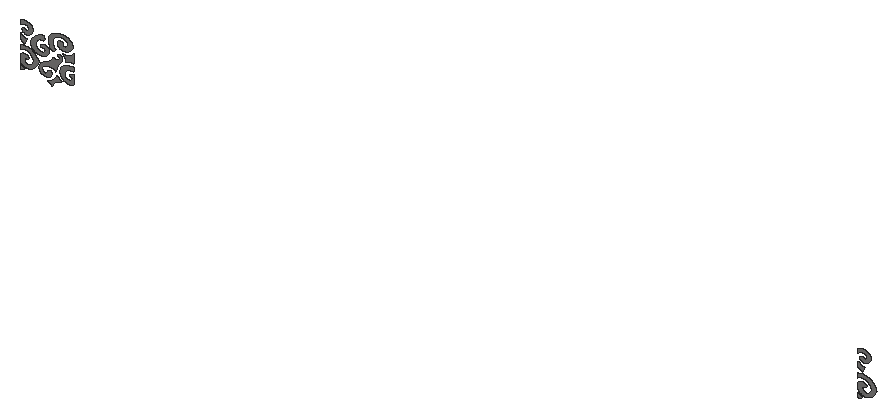
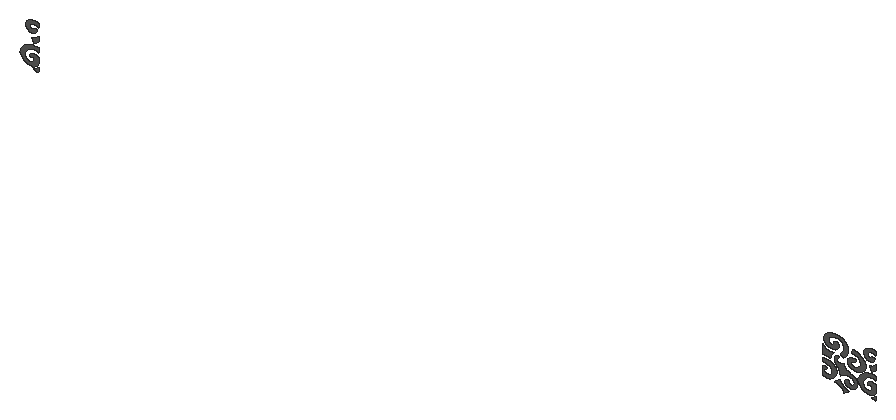
# SketchUp Ruby script. Lengths in inches.
U = 1.inch
M = Sketchup.active_model
def pt(a) = Geom::Point3d.new(a.map { |v| v * U })
def face(e, loops, mat)
  f = e.add_face(loops[0].map { |a| pt(a) })
  loops[1..].each { |l| e.add_face(l.map { |a| pt(a) }).erase! }
  f.material = f.back_material = mat if mat
  f
end
# faces: each face lists its corners as indices into pts; further lists are holes
def faces(e, pts, list, mat = nil) = list.each { |f| face(e, (f[0].is_a?(Array) ? f : [f]).map { |l| l.map { |i| pts[i] } }, mat) }
# xy, xz, yz: faces in a plane at the given z, y or x. An outline is a flat list of corners, or four numbers for a rectangle; further outlines are holes
def ring(l) = l.size == 4 ? [[l[0], l[1]], [l[2], l[1]], [l[2], l[3]], [l[0], l[3]]] : l.each_slice(2).to_a
def flat(e, list, mat, &to3) = list.each { |f| face(e, (f[0].is_a?(Array) ? f : [f]).map { |l| ring(l).map { |u, v| to3.(u, v) } }, mat) }
def xy(e, z, list, mat = nil) = flat(e, list, mat) { |x, y| [x, y, z] }
def xz(e, y, list, mat = nil) = flat(e, list, mat) { |x, z| [x, y, z] }
def yz(e, x, list, mat = nil) = flat(e, list, mat) { |y, z| [x, y, z] }
def lines(e, pts, list) = list.each { |a, b| e.add_line(pt(pts[a]), pt(pts[b])) }
# prism: a flat outline (further loops are holes) pulled along v
def prism(e, loops, v, mat = nil)
  f = face(e, loops, mat); d = Geom::Vector3d.new(v.map { |x| x * U })
  f.pushpull(f.normal.samedirection?(d) ? d.length : -d.length)
end
def box(e, o, s, mat = nil) = prism(e, [[o, [o[0] + s[0], o[1], o[2]], [o[0] + s[0], o[1] + s[1], o[2]], [o[0], o[1] + s[1], o[2]]]], [0, 0, s[2]], mat)
def at(x, y, z, deg = 0) = Geom::Transformation.translation(pt([x, y, z])) * Geom::Transformation.rotation(ORIGIN, Z_AXIS, deg.degrees)
def axes(o, x, y, z) = Geom::Transformation.new([*x, 0, *y, 0, *z, 0, *pt(o).to_a, 1])
def part(name) = M.definitions.add(name)
# library, detail: a bought-in or finely detailed component or shape, given as its bounding box
def library(name, o, s) = part(name).tap { |d| box(d.entities, o, s) }
def detail(e, o, s) = box(e.add_group.entities, o, s)
def put(e, d, t, mat = nil) = e.add_instance(d, t).tap { |i| i.material = mat if mat }
def group(e, t, mat = nil) = e.add_group.tap { |g| g.transformation = t; g.material = mat if mat }.entities
root = M.entities
M.materials.add("[0043_SaddleBrown]4").color = [124, 123, 122]
xz(root,589.17,[[416.17,173.83,415.69,174.24,415.1875,174.64,414.66,175.02,414.12,175.39,413.5625,175.74,412.98,176.08,412.39,176.4,411.78,176.71,411.15,177,410.51,177.27,409.85,177.53,409.1875,177.77,410.75,178.34,412.25,178.99,413.6875,179.72,415.05,180.52,416.32,181.39,417.51,182.32,418.6,183.31,419.6,184.35,420.48,185.44,421.26,186.58,421.93,187.75,422.47,188.95,423.02,188.49,423.58,188.03,424.74,187.15,425.33,186.72,425.93,186.29,426.54,185.87,427.16,185.46,427.79,185.06,428.43,184.66,429.07,184.27,429.73,183.89,428.07,183.57,426.46,183.14,424.92,182.59,423.45,181.94,422.09,181.19,420.83,180.35,419.7,179.42,418.69,178.41,417.83,177.34,417.12,176.21,416.56,175.04],[367.98,179.89,367.98,185.26,368.39,184.92,368.83,184.6,369.28,184.3,369.76,184.01,370.25,183.73,370.76,183.47,371.28,183.23,371.82,183,372.37,182.79,372.93,182.6,373.51,182.42,374.09,182.27,373.71,181.9375,373.3,181.63,372.86,181.34,372.39,181.07,371.9,180.83,371.38,180.61,370.85,180.42,370.3,180.26,369.73,180.12,369.15,180.02,368.57,179.9375],[1618.6,179.89,1618.6,185.26,1619.02,184.92,1619.45,184.6,1619.91,184.3,1620.38,184.01,1620.875,183.73,1621.38,183.47,1621.9,183.23,1622.44,183,1622.99,182.79,1623.56,182.6,1624.13,182.42,1624.72,182.27,1624.34,181.9375,1623.92,181.63,1623.48,181.34,1623.02,181.07,1622.52,180.83,1622.01,180.61,1621.47,180.42,1620.92,180.26,1620.36,180.12,1619.78,180.02,1619.19,179.9375],[405.4,183.24,403.96,183.36,402.58,183.65,401.26,184.08,400.05,184.65,398.98,185.34,398.07,186.15,397.33,187.04,396.79,188.01,396.47,189.02,396.36,190.0625,396.24,191.26,396.31,192.46,396.54,193.65,396.94,194.8125,397.51,195.9375,398.24,197.02,399.12,198.04,400.14,198.99,401.29,199.85,402.56,200.63,403.93,201.31,405.4,201.88,406.79,202.4,408.12,202.99,409.39,203.65,410.6,204.37,411.73,205.15,412.78,205.98,413.74,206.87,414.62,207.81,415.4,208.78,416.09,209.8,416.67,210.85,417.15,211.92,417.83,211.55,418.57,211.25,419.36,211.03,420.18,210.88,421.03,210.82,421.88,210.84,422.72,210.9375,423.53,211.12,424.3,211.38,425.01,211.72,425.65,212.12,426.22,212.58,426.42,212.95,426.57,213.33,426.65,213.73,426.68,214.13,426.64,214.53,426.53,214.92,426.37,215.3,426.15,215.67,425.875,216.02,425.54,216.34,425.17,216.63,424.75,216.89,424.52,217.04,424.33,217.23,424.2,217.43,424.13,217.65,424.12,217.875,424.17,218.1,424.28,218.3125,424.44,218.5,424.65,218.67,424.91,218.8,425.19,218.9,425.5,218.95,426.05,218.98,426.61,218.95,427.15,218.86,427.68,218.72,428.16,218.52,428.61,218.28,429,217.99,429.33,217.67,429.6,217.3125,429.79,216.9375,429.91,216.54,429.94,216.14,430.16,215.47,430.3,214.79,430.38,214.11,430.39,213.42,430.32,212.73,430.19,212.05,429.99,211.38,429.73,210.72,429.39,210.08,428.99,209.45,428.54,208.85,428.02,208.27,427.08,207.26,426.21,206.23,425.41,205.16,424.67,204.07,424,202.95,423.41,201.82,422.88,200.67,422.43,199.5,422.05,198.32,421.75,197.12,421.52,195.92,421.37,194.71,420.4,195.61,419.28,196.41,418.03,197.09,416.66,197.66,415.2,198.09,413.68,198.375,412.12,198.52,410.54,198.52,408.98,198.37,407.46,198.07,406.01,197.63,404.64,197.0625,403.67,196.53,402.8,195.9,402.05,195.2,401.43,194.44,400.95,193.625,400.625,192.77,400.45,191.9,400.43,191.01,400.57,190.14,400.87,189.28,401.32,188.46,401.91,187.68,402.45,187.38,403.06,187.15,403.7,186.98,404.37,186.89,405.05,186.87,405.73,186.92,406.39,187.04,407.02,187.24,407.6,187.5,408.12,187.82,408.57,188.1875,408.9375,188.6,408.82,188.9,408.73,189.2,408.68,189.5,408.66,189.81,408.67,190.12,408.72,190.42,408.8,190.72,408.91,191.02,409.06,191.31,409.24,191.59,409.45,191.86,409.68,192.11,409.91,192.31,410.1875,192.48,410.49,192.61,410.82,192.71,411.17,192.77,411.53,192.79,411.89,192.77,412.23,192.71,412.57,192.61,412.87,192.48,413.14,192.31,413.375,192.11,414.05,191.31,414.52,190.43,414.78,189.51,414.8125,188.57,414.625,187.63,414.22,186.74,413.6,185.91,412.8,185.17,411.84,184.53,410.74,184.03,409.53,183.66,408.26,183.45,406.84,183.27],[378.13,184.38,376.97,184.54,375.83,184.78,374.74,185.09,373.6875,185.48,372.69,185.94,371.76,186.47,370.91,187.05,370.13,187.69,369.45,188.38,368.86,189.12,368.36,189.89,367.98,190.7,367.98,198.78,368.51,199.6875,369.28,200.5,370.27,201.17,371.43,201.69,372.71,202.03,374.05,202.17,375.42,202.12,376.73,201.86,377.95,201.42,379.01,200.8,379.88,200.05,380.52,199.18,380.62,198.97,380.67,198.75,380.67,198.53,380.63,198.32,380.55,198.1,380.42,197.9,380.26,197.72,380.06,197.55,379.82,197.41,379.57,197.3,379.29,197.21,378.99,197.15,378.26,197.24,377.53,197.23,376.81,197.13,376.125,196.93,375.5,196.64,374.97,196.28,374.53,195.85,374.22,195.37,374.03,194.85,373.97,194.32,374.06,193.8,374.27,193.29,374.45,192.63,374.78,192,375.24,191.41,375.82,190.88,376.51,190.43,377.28,190.06,378.13,189.78,379.03,189.6,379.96,189.53,380.89,189.5625,381.81,189.7,382.68,189.9375,384.03,190.72,385.22,191.64,386.22,192.67,387,193.79,387.5625,194.98,387.88,196.21,387.95,197.47,387.78,198.72,387.36,199.93,386.71,201.1,385.84,202.18,384.76,203.17,384.32,203.82,383.81,204.45,383.22,205.04,382.58,205.59,381.87,206.1,381.1,206.57,380.28,206.99,379.42,207.37,378.51,207.68,377.57,207.94,376.61,208.15,375.625,208.3,374.92,208.36,374.22,208.375,373.51,208.35,372.8125,208.28,372.12,208.17,371.45,208.02,370.79,207.83,370.16,207.6,369.5625,207.33,368.99,207.03,368.46,206.69,367.98,206.32,367.98,211.9,370.12,212.41,372.34,212.74,374.59,212.875,376.85,212.8125,379.09,212.56,381.26,212.11,383.35,211.48,385.3125,210.67,387.13,209.7,388.77,208.58,390.22,207.33,391.45,205.96,393.12,203.92,394.27,201.7,394.89,199.375,394.93,197.01,394.41,194.67,393.34,192.43,391.75,190.36,389.6875,188.51,387.21,186.95,384.41,185.72,381.35,184.86],
  [1628.75,184.38,1627.59,184.54,1626.46,184.78,1625.36,185.09,1624.3125,185.48,1623.32,185.94,1622.39,186.47,1621.53,187.05,1620.76,187.69,1620.07,188.38,1619.48,189.12,1618.99,189.89,1618.6,190.7,1618.6,198.78,1619.13,199.6875,1619.91,200.5,1620.89,201.17,1622.05,201.69,1623.33,202.03,1624.68,202.17,1626.04,202.12,1627.36,201.86,1628.57,201.42,1629.64,200.8,1630.51,200.05,1631.15,199.18,1631.24,198.97,1631.29,198.75,1631.3,198.53,1631.26,198.32,1631.17,198.1,1631.05,197.9,1630.88,197.72,1630.68,197.55,1630.45,197.41,1630.19,197.3,1629.91,197.21,1629.62,197.15,1628.89,197.24,1628.15,197.23,1627.43,197.13,1626.75,196.93,1626.13,196.64,1625.59,196.28,1625.16,195.85,1624.84,195.37,1624.65,194.85,1624.6,194.32,1624.68,193.8,1624.9,193.29,1625.08,192.63,1625.4,192,1625.86,191.41,1626.44,190.88,1627.13,190.43,1627.91,190.06,1628.76,189.78,1629.66,189.6,1630.59,189.53,1631.52,189.5625,1632.43,189.7,1633.3,189.9375,1634.66,190.72,1635.85,191.64,1636.84,192.67,1637.63,193.79,1638.1875,194.98,1638.5,196.21,1638.58,197.47,1638.4,198.72,1637.99,199.93,1637.33,201.1,1636.46,202.18,1635.38,203.17,1634.94,203.82,1634.43,204.45,1633.85,205.04,1633.2,205.59,1632.49,206.1,1631.72,206.57,1630.9,206.99,1630.04,207.37,1629.14,207.68,1628.2,207.94,1627.23,208.15,1626.25,208.3,1625.55,208.36,1624.84,208.375,1624.14,208.35,1623.4375,208.28,1622.75,208.17,1622.07,208.02,1621.42,207.83,1620.79,207.6,1620.1875,207.33,1619.62,207.03,1619.09,206.69,1618.6,206.32,1618.6,211.9,1620.75,212.41,1622.96,212.74,1625.22,212.875,1627.48,212.8125,1629.71,212.56,1631.89,212.11,1633.97,211.48,1635.9375,210.67,1637.76,209.7,1639.4,208.58,1640.85,207.33,1642.07,205.96,1643.74,203.92,1644.9,201.7,1645.51,199.375,1645.56,197.01,1645.03,194.67,1643.96,192.43,1642.37,190.36,1640.3125,188.51,1637.84,186.95,1635.03,185.72,1631.97,184.86],[440.93,185,439.57,185.0625,438.23,185.24,436.9375,185.54,435.7,185.94,434.55,186.46,433.49,187.07,432.59,187.69,431.76,188.36,430.99,189.0625,430.28,189.8,429.65,190.57,429.09,191.375,428.61,192.2,428.2,193.05,427.875,193.92,427.63,194.79,427.47,195.68,427.39,196.58,427.5,198.46,428.01,200.32,428.9,202.09,430.15,203.75,431.73,205.26,433.61,206.58,435.74,207.67,438.08,208.53,440.57,209.12,443.15,209.4375,445.77,209.47,448.37,209.22,448.37,204.51,446.14,204.57,443.93,204.34,441.81,203.84,439.84,203.08,438.08,202.09,436.59,200.89,435.41,199.53,434.58,198.03,434.12,196.46,434.05,194.85,434.37,193.26,435.0625,191.73,435.86,191.08,436.81,190.54,437.88,190.15,439.04,189.91,440.24,189.83,441.45,189.91,442.6,190.16,443.68,190.55,444.625,191.09,445.42,191.75,446.03,192.5,446.43,193.32,446.5,193.65,446.49,193.99,446.41,194.32,446.24,194.64,446,194.93,445.7,195.19,445.34,195.4,444.9375,195.57,444.5,195.6875,444.04,195.75,443.57,195.75,443.11,195.7,442.87,195.77,442.64,195.87,442.43,195.98,442.23,196.11,442.06,196.25,441.9,196.41,441.78,196.58,441.67,196.75,441.6,196.93,441.55,197.12,441.53,197.3125,441.54,197.5,441.9,197.89,442.34,198.24,442.84,198.54,443.39,198.8,443.98,199,444.6,199.14,445.24,199.22,445.89,199.24,446.54,199.19,447.18,199.09,447.79,198.93,448.37,198.7,448.37,187.07,447.3,186.46,446.15,185.94,444.91,185.54,443.62,185.24,442.28,185.0625],[398.82,208.61,396.48,208.71,394.2,209.07,392.02,209.68,390,210.53,388.1875,211.6,386.63,212.86,385.36,214.28,384.42,215.82,383.82,217.45,383.58,219.125,383.71,220.81,384.2,222.46,384.75,224.06,385.51,225.62,386.46,227.12,387.6,228.55,388.91,229.9,390.4,231.16,392.03,232.31,393.81,233.35,395.71,234.27,397.72,235.06,399.82,235.71,402,236.22,402.41,235.77,402.78,235.31,403.09,234.82,403.35,234.32,403.5625,233.81,403.72,233.28,403.82,232.75,403.86,232.22,403.85,231.68,403.79,231.15,403.67,230.62,403.49,230.1,402.14,230.21,400.78,230.19,399.44,230.04,398.13,229.75,396.9,229.33,395.76,228.8,394.73,228.16,393.83,227.42,393.09,226.6,392.51,225.71,392.1,224.77,391.875,223.8,391.51,222.89,391.28,221.95,391.1875,221,391.24,220.05,391.43,219.11,391.77,218.19,392.23,217.3,392.83,216.45,393.55,215.65,394.38,214.91,395.32,214.24,396.35,213.65,397.31,213.25,398.35,212.99,399.45,212.875,400.55,212.91,401.625,213.1,402.63,213.43,403.54,213.89,404.3,214.46,404.9,215.13,405.32,215.875,405.53,216.66,405.53,217.45,405.45,217.85,405.29,218.23,405.06,218.59,404.76,218.92,404.4,219.23,403.99,219.49,403.53,219.71,403.04,219.89,402.51,220.01,401.97,220.09,401.42,220.1,400.87,220.07,400.3,220.05,399.73,220.13,399.21,220.3,398.75,220.55,398.38,220.86,398.12,221.23,397.99,221.63,397.98,222.05,398.11,222.45,398.36,222.83,398.72,223.15,399.17,223.4,400.41,223.84,401.75,224.12,403.14,224.21,404.52,224.12,405.86,223.85,407.1,223.4,408.22,222.81,409.16,222.07,409.91,221.23,410.43,220.3,410.71,219.32,410.73,218.32,410.79,217.11,410.61,215.9,410.21,214.72,409.58,213.6,408.75,212.54,407.73,211.58,406.53,210.73,405.18,210.01,403.7,209.42,402.13,208.99,400.49,208.72],[436.38,213.07,436.28,213.85,436.12,214.62,435.91,215.39,435.64,216.14,435.32,216.89,434.95,217.625,434.53,218.34,434.05,219.05,433.53,219.73,432.96,220.4,432.34,221.04,431.68,221.66,433.34,221.55,435,221.5625,436.65,221.7,438.27,221.96,439.85,222.33,441.36,222.82,442.8,223.41,444.15,224.11,445.39,224.91,446.52,225.79,447.51,226.75,448.37,227.78,448.37,215.23,447.33,215.21,446.29,215.16,445.26,215.08,444.23,214.98,443.21,214.84,442.2,214.67,441.19,214.47,440.2,214.25,439.22,213.99,438.26,213.71,437.3125,213.41],[375.32,216.375,374.62,216.63,373.94,216.91,373.26,217.2,372.61,217.52,371.97,217.84,371.34,218.1875,370.73,218.54,370.14,218.92,369.57,219.31,369.02,219.71,368.49,220.125,367.98,220.56,367.98,227.67,368.5,227.04,369.09,226.43,369.74,225.86,370.46,225.34,371.24,224.85,372.07,224.42,372.94,224.03,373.86,223.7,374.81,223.42,375.78,223.2,376.78,223.04,377.8,222.93,377.38,222.44,377,221.9375,376.65,221.42,376.35,220.89,376.08,220.35,375.85,219.79,375.66,219.23,375.51,218.67,375.4,218.1,375.33,217.52,375.3,216.95],
  [1625.94,216.375,1625.25,216.63,1624.56,216.91,1623.89,217.2,1623.23,217.52,1622.59,217.84,1621.97,218.1875,1621.36,218.54,1620.77,218.92,1620.2,219.31,1619.64,219.71,1619.11,220.125,1618.6,220.56,1618.6,227.67,1619.12,227.04,1619.71,226.43,1620.37,225.86,1621.09,225.34,1621.86,224.85,1622.69,224.42,1623.57,224.03,1624.48,223.7,1625.43,223.42,1626.41,223.2,1627.41,223.04,1628.43,222.93,1628.01,222.44,1627.625,221.9375,1627.28,221.42,1626.97,220.89,1626.7,220.35,1626.47,219.79,1626.28,219.23,1626.13,218.67,1626.02,218.1,1625.96,217.52,1625.93,216.95],[415.77,220.74,414.64,221.82,413.63,222.95,412.74,224.13,411.98,225.36,411.34,226.63,410.84,227.92,410.47,229.24,410.24,230.58,410.15,231.92,410.19,233.27,410.375,234.61,410.7,235.94,411.23,237.37,411.96,238.75,412.88,240.07,413.98,241.32,415.26,242.48,416.69,243.55,418.26,244.5,419.97,245.33,421.77,246.03,423.67,246.59,425.64,247.02,427.66,247.29,429.86,247.4,432.06,247.29,434.23,246.97,436.31,246.4375,438.27,245.71,440.07,244.79,441.69,243.71,443.08,242.47,444.23,241.12,445.11,239.66,445.71,238.125,446.02,236.55,446.01,235.18,445.73,233.83,445.18,232.52,444.36,231.29,443.31,230.15,442.04,229.14,440.57,228.27,438.94,227.57,437.19,227.04,435.35,226.71,433.47,226.57,431.57,226.63,430.1,226.85,428.69,227.24,427.4,227.79,426.24,228.48,425.26,229.3,424.48,230.23,423.92,231.23,423.59,232.29,423.51,233.37,423.68,234.45,424.09,235.49,424.73,236.47,425.24,236.87,425.86,237.18,426.55,237.39,427.29,237.5,428.04,237.49,428.77,237.375,429.46,237.15,430.07,236.83,430.57,236.43,430.95,235.96,431.18,235.44,431.07,235.09,431.01,234.73,431.01,234.37,431.0625,234.01,431.17,233.65,431.34,233.3125,431.55,232.98,431.82,232.68,432.13,232.39,432.48,232.13,432.875,231.91,433.3,231.71,434.31,231.82,435.29,232.03,436.21,232.35,437.05,232.77,437.79,233.28,438.41,233.86,438.91,234.5,439.26,235.19,439.46,235.91,439.5,236.65,439.39,237.38,439.12,238.09,438.37,239.28,437.36,240.36,436.11,241.3,434.67,242.08,433.0625,242.67,431.34,243.07,429.55,243.25,427.75,243.21,425.98,242.96,424.29,242.5,422.73,241.84,421.35,241,419.9,239.82,418.67,238.51,417.7,237.1,416.99,235.6,416.5625,234.06,416.42,232.48,416.5625,230.91,416.99,229.36,417.7,227.86,418.67,226.45,419.9,225.14,421.35,223.96,420.98,223.61,420.6,223.28,420.19,222.95,419.77,222.65,419.33,222.35,418.86,222.07,418.38,221.81,417.89,221.5625,417.38,221.33,416.85,221.12,416.32,220.92],[377.83,229.18,376.55,229.23,375.3,229.45,374.13,229.84,373.09,230.38,372.21,231.06,371.52,231.84,371.04,232.7,370.8,233.61,370.71,233.96,370.72,234.32,370.82,234.67,371.01,235,371.29,235.29,371.65,235.54,372.06,235.74,372.52,235.875,373,235.94,373.5,235.94,373.99,235.87,374.44,235.73,374.71,235.48,375,235.24,375.31,235.01,375.64,234.8,375.98,234.6,376.35,234.42,376.72,234.26,377.12,234.11,377.52,233.98,377.93,233.87,378.36,233.78,378.78,233.71,379.35,234.05,379.85,234.45,380.28,234.89,380.625,235.36,380.9,235.86,381.08,236.375,381.17,236.91,381.17,237.44,381.08,237.97,380.9,238.49,380.64,238.99,380.29,239.46,379.5625,240.18,378.68,240.79,377.66,241.29,376.54,241.65,375.36,241.875,374.13,241.95,372.91,241.875,371.72,241.65,370.6,241.29,369.59,240.79,368.7,240.18,367.98,239.46,367.98,244.71,368.85,245.16,369.78,245.55,370.76,245.87,371.78,246.125,372.83,246.3,373.9,246.41,374.97,246.4375,376.05,246.39,377.11,246.27,378.15,246.08,379.17,245.8125,380.14,245.48,381.83,244.68,383.33,243.71,384.59,242.57,385.58,241.3,386.28,239.93,386.66,238.5,386.72,237.04,386.46,235.6,385.88,234.2,384.99,232.89,383.83,231.7,382.42,230.65,381.4375,230.05,380.32,229.6,379.1,229.3],[1628.45,229.18,1627.17,229.23,1625.92,229.45,1624.76,229.84,1623.72,230.38,1622.83,231.06,1622.14,231.84,1621.67,232.7,1621.43,233.61,1621.34,233.96,1621.34,234.32,1621.45,234.67,1621.64,235,1621.92,235.29,1622.27,235.54,1622.68,235.74,1623.14,235.875,1623.63,235.94,1624.125,235.94,1624.61,235.87,1625.07,235.73,1625.34,235.48,1625.625,235.24,1625.93,235.01,1626.26,234.8,1626.61,234.6,1626.97,234.42,1627.35,234.26,1627.74,234.11,1628.14,233.98,1628.56,233.87,1628.98,233.78,1629.41,233.71,1629.97,234.05,1630.47,234.45,1630.9,234.89,1631.25,235.36,1631.52,235.86,1631.7,236.375,1631.79,236.91,1631.8,237.44,1631.71,237.97,1631.53,238.49,1631.26,238.99,1630.91,239.46,1630.1875,240.18,1629.3,240.79,1628.29,241.29,1627.17,241.65,1625.98,241.875,1624.76,241.95,1623.53,241.875,1622.35,241.65,1621.23,241.29,1620.21,240.79,1619.33,240.18,1618.6,239.46,1618.6,244.71,1619.48,245.16,1620.41,245.55,1621.39,245.87,1622.41,246.125,1623.45,246.3,1624.52,246.41,1625.6,246.4375,1626.67,246.39,1627.74,246.27,1628.78,246.08,1629.79,245.8125,1630.76,245.48,1632.46,244.68,1633.96,243.71,1635.22,242.57,1636.21,241.3,1636.9,239.93,1637.29,238.5,1637.35,237.04,1637.08,235.6,1636.5,234.2,1635.62,232.89,1634.46,231.7,1633.04,230.65,1632.0625,230.05,1630.95,229.6,1629.73,229.3]],"[0043_SaddleBrown]4")
p = [[431.27,589.17,234.9],[431.18,589.17,235.44],[367.98,589.17,176.23],[367.98,589.17,179.89],[1618.6,589.17,176.23],[1618.6,589.17,179.89]]
lines(root,p,[[0,1],[2,3],[4,5]])
